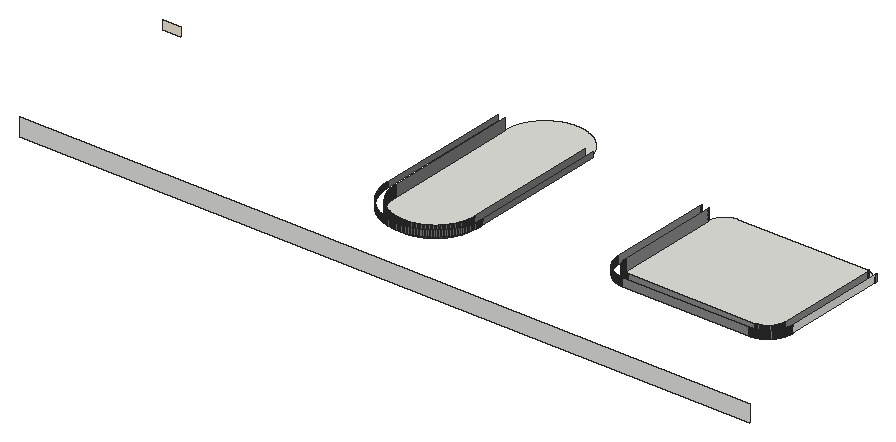
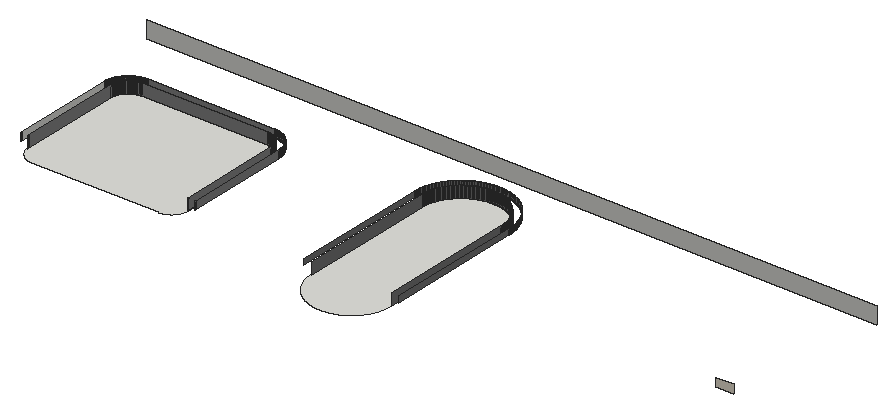
# SketchUp Ruby script. Lengths in inches.
U = 1.inch
M = Sketchup.active_model
def pt(a) = Geom::Point3d.new(a.map { |v| v * U })
def face(e, loops, mat)
  f = e.add_face(loops[0].map { |a| pt(a) })
  loops[1..].each { |l| e.add_face(l.map { |a| pt(a) }).erase! }
  f.material = f.back_material = mat if mat
  f
end
# faces: each face lists its corners as indices into pts; further lists are holes
def faces(e, pts, list, mat = nil) = list.each { |f| face(e, (f[0].is_a?(Array) ? f : [f]).map { |l| l.map { |i| pts[i] } }, mat) }
# xy, xz, yz: faces in a plane at the given z, y or x. An outline is a flat list of corners, or four numbers for a rectangle; further outlines are holes
def ring(l) = l.size == 4 ? [[l[0], l[1]], [l[2], l[1]], [l[2], l[3]], [l[0], l[3]]] : l.each_slice(2).to_a
def flat(e, list, mat, &to3) = list.each { |f| face(e, (f[0].is_a?(Array) ? f : [f]).map { |l| ring(l).map { |u, v| to3.(u, v) } }, mat) }
def xy(e, z, list, mat = nil) = flat(e, list, mat) { |x, y| [x, y, z] }
def xz(e, y, list, mat = nil) = flat(e, list, mat) { |x, z| [x, y, z] }
def yz(e, x, list, mat = nil) = flat(e, list, mat) { |y, z| [x, y, z] }
def lines(e, pts, list) = list.each { |a, b| e.add_line(pt(pts[a]), pt(pts[b])) }
# prism: a flat outline (further loops are holes) pulled along v
def prism(e, loops, v, mat = nil)
  f = face(e, loops, mat); d = Geom::Vector3d.new(v.map { |x| x * U })
  f.pushpull(f.normal.samedirection?(d) ? d.length : -d.length)
end
def box(e, o, s, mat = nil) = prism(e, [[o, [o[0] + s[0], o[1], o[2]], [o[0] + s[0], o[1] + s[1], o[2]], [o[0], o[1] + s[1], o[2]]]], [0, 0, s[2]], mat)
def at(x, y, z, deg = 0) = Geom::Transformation.translation(pt([x, y, z])) * Geom::Transformation.rotation(ORIGIN, Z_AXIS, deg.degrees)
def axes(o, x, y, z) = Geom::Transformation.new([*x, 0, *y, 0, *z, 0, *pt(o).to_a, 1])
def part(name) = M.definitions.add(name)
# library, detail: a bought-in or finely detailed component or shape, given as its bounding box
def library(name, o, s) = part(name).tap { |d| box(d.entities, o, s) }
def detail(e, o, s) = box(e.add_group.entities, o, s)
def put(e, d, t, mat = nil) = e.add_instance(d, t).tap { |i| i.material = mat if mat }
def group(e, t, mat = nil) = e.add_group.tap { |g| g.transformation = t; g.material = mat if mat }.entities
root = M.entities
M.materials.add("0027 AP L140 CRUSHED ICE").color = [241, 233, 217]
M.materials.add("[Slate Light Tile]").color = [119, 119, 119]
M.materials.add("[Stone Coursed Rough]").color = [137, 137, 137]
xy(root,-3,[[189,27,189.55,27.01,190.1,27.03,190.65,27.06,191.2,27.12,191.74,27.18,192.29,27.26,192.83,27.35,193.37,27.46,193.9,27.58,194.44,27.72,194.96,27.86,195.49,28.03,196.01,28.2,196.53,28.39,197.04,28.6,197.54,28.82,198.04,29.05,198.53,29.29,199.02,29.54,199.5,29.8125,199.97,30.09,200.4375,30.39,200.89,30.69,201.34,31.01,201.78,31.34,202.22,31.68,202.64,32.03,203.05,32.39,203.46,32.77,203.85,33.15,204.23,33.54,204.61,33.95,204.97,34.36,205.32,34.78,205.66,35.22,205.99,35.66,206.31,36.11,206.61,36.5625,206.91,37.03,207.1875,37.5,207.46,37.98,207.71,38.47,207.95,38.96,208.18,39.46,208.4,39.96,208.61,40.47,208.8,40.99,208.97,41.51,209.14,42.04,209.28,42.56,209.42,43.1,209.54,43.63,209.65,44.17,209.74,44.71,209.82,45.26,209.88,45.8,209.94,46.35,209.97,46.9,209.99,47.45,210,48,210,120,209.99,120.55,209.97,121.1,209.94,121.65,209.88,122.2,209.82,122.74,209.74,123.29,209.65,123.83,209.54,124.37,209.42,124.9,209.28,125.44,209.14,125.96,208.97,126.49,208.8,127.01,208.61,127.53,208.4,128.04,208.18,128.54,207.95,129.04,207.71,129.53,207.46,130.02,207.1875,130.5,206.91,130.97,206.61,131.4375,206.31,131.89,205.99,132.34,205.66,132.78,205.32,133.22,204.97,133.64,204.61,134.05,204.23,134.46,203.85,134.85,203.46,135.23,203.05,135.61,202.64,135.97,202.22,136.32,201.78,136.66,201.34,136.99,200.89,137.31,200.4375,137.61,199.97,137.91,199.5,138.1875,199.02,138.46,198.53,138.71,198.04,138.95,197.54,139.18,197.04,139.4,196.53,139.61,196.01,139.8,195.49,139.97,194.96,140.14,194.44,140.28,193.9,140.42,193.37,140.54,192.83,140.65,192.29,140.74,191.74,140.82,191.2,140.88,190.65,140.94,190.1,140.97,189.55,140.99,189,141,188.45,140.99,187.9,140.97,187.35,140.94,186.8,140.88,186.26,140.82,185.71,140.74,185.17,140.65,184.63,140.54,184.1,140.42,183.56,140.28,183.04,140.14,182.51,139.97,181.99,139.8,181.47,139.61,180.96,139.4,180.46,139.18,179.96,138.95,179.47,138.71,178.98,138.46,178.5,138.1875,178.03,137.91,177.5625,137.61,177.11,137.31,176.66,136.99,176.22,136.66,175.78,136.32,175.36,135.97,174.95,135.61,174.54,135.23,174.15,134.85,173.77,134.46,173.39,134.05,173.03,133.64,172.68,133.22,172.34,132.78,172.01,132.34,171.69,131.89,171.39,131.4375,171.09,130.97,170.8125,130.5,170.54,130.02,170.29,129.53,170.05,129.04,169.82,128.54,169.6,128.04,169.39,127.53,169.2,127.01,169.03,126.49,168.86,125.96,168.72,125.44,168.58,124.9,168.46,124.37,168.35,123.83,168.26,123.29,168.18,122.74,168.12,122.2,168.06,121.65,168.03,121.1,168.01,120.55,168,120,168,48,168.01,47.45,168.03,46.9,168.06,46.35,168.12,45.8,168.18,45.26,168.26,44.71,168.35,44.17,168.46,43.63,168.58,43.1,168.72,42.56,168.86,42.04,169.03,41.51,169.2,40.99,169.39,40.47,169.6,39.96,169.82,39.46,170.05,38.96,170.29,38.47,170.54,37.98,170.8125,37.5,171.09,37.03,171.39,36.5625,171.69,36.11,172.01,35.66,172.34,35.22,172.68,34.78,173.03,34.36,173.39,33.95,173.77,33.54,174.15,33.15,174.54,32.77,174.95,32.39,175.36,32.03,175.78,31.68,176.22,31.34,176.66,31.01,177.11,30.69,177.5625,30.39,178.03,30.09,178.5,29.8125,178.98,29.54,179.47,29.29,179.96,29.05,180.46,28.82,180.96,28.6,181.47,28.39,181.99,28.2,182.51,28.03,183.04,27.86,183.56,27.72,184.1,27.58,184.63,27.46,185.17,27.35,185.71,27.26,186.26,27.18,186.8,27.12,187.35,27.06,187.9,27.03,188.45,27.01]])
xy(root,-2,[[290.72,48,357.28,48,357.57,48.02,357.85,48.04,358.13,48.07,358.41,48.11,358.6875,48.16,358.96,48.22,359.24,48.28,359.78,48.44,360.05,48.53,360.3125,48.63,360.57,48.74,361.09,48.98,361.34,49.11,361.58,49.25,361.82,49.4,362.06,49.56,362.29,49.72,362.52,49.89,362.74,50.07,362.95,50.25,363.16,50.4375,363.36,50.64,363.5625,50.84,363.75,51.05,363.93,51.26,364.11,51.48,364.28,51.71,364.44,51.94,364.6,52.18,364.75,52.42,364.89,52.66,365.02,52.91,365.26,53.43,365.37,53.6875,365.47,53.95,365.56,54.22,365.72,54.76,365.78,55.04,365.84,55.3125,365.89,55.59,365.93,55.87,365.96,56.15,365.98,56.43,366,56.72,366,111.28,365.98,111.57,365.96,111.85,365.93,112.13,365.89,112.41,365.84,112.6875,365.78,112.96,365.72,113.24,365.56,113.78,365.47,114.05,365.37,114.3125,365.26,114.57,365.02,115.09,364.89,115.34,364.75,115.58,364.6,115.82,364.44,116.06,364.28,116.29,364.11,116.52,363.93,116.74,363.75,116.95,363.5625,117.16,363.36,117.36,363.16,117.5625,362.95,117.75,362.74,117.93,362.52,118.11,362.29,118.28,362.06,118.44,361.82,118.6,361.58,118.75,361.34,118.89,361.09,119.02,360.57,119.26,360.3125,119.37,360.05,119.47,359.78,119.56,359.24,119.72,358.96,119.78,358.6875,119.84,358.41,119.89,358.13,119.93,357.85,119.96,357.57,119.98,357.28,120,290.72,120,290.43,119.98,290.15,119.96,289.87,119.93,289.59,119.89,289.3125,119.84,289.04,119.78,288.76,119.72,288.22,119.56,287.95,119.47,287.6875,119.37,287.43,119.26,286.91,119.02,286.66,118.89,286.42,118.75,286.18,118.6,285.94,118.44,285.71,118.28,285.48,118.11,285.26,117.93,285.05,117.75,284.84,117.5625,284.64,117.36,284.4375,117.16,284.25,116.95,284.07,116.74,283.89,116.52,283.72,116.29,283.56,116.06,283.4,115.82,283.25,115.58,283.11,115.34,282.98,115.09,282.74,114.57,282.63,114.3125,282.53,114.05,282.44,113.78,282.28,113.24,282.22,112.96,282.16,112.6875,282.11,112.41,282.07,112.13,282.04,111.85,282.02,111.57,282,111.28,282,56.72,282.02,56.43,282.04,56.15,282.07,55.87,282.11,55.59,282.16,55.3125,282.22,55.04,282.28,54.76,282.44,54.22,282.53,53.95,282.63,53.6875,282.74,53.43,282.98,52.91,283.11,52.66,283.25,52.42,283.4,52.18,283.56,51.94,283.72,51.71,283.89,51.48,284.07,51.26,284.25,51.05,284.4375,50.84,284.64,50.64,284.84,50.4375,285.05,50.25,285.26,50.07,285.48,49.89,285.71,49.72,285.94,49.56,286.18,49.4,286.42,49.25,286.66,49.11,286.91,48.98,287.43,48.74,287.6875,48.63,287.95,48.53,288.22,48.44,288.76,48.28,289.04,48.22,289.3125,48.16,289.59,48.11,289.87,48.07,290.15,48.04,290.43,48.02]])
xz(root,0,[[9,-9,393,0]])
xz(root,44,[[291,0,357,4]],"[Stone Coursed Rough]")
xz(root,48,[[290.72,-2,291,4],[291,-2,357,4],[357,-2,357.28,4]],"[Stone Coursed Rough]")
xz(root,94,[[9,0,18,4.5]],"0027 AP L140 CRUSHED ICE")
yz(root,164,[[48,0,120,3]],"[Slate Light Tile]")
yz(root,168,[[48,-3,120,3]],"[Slate Light Tile]")
yz(root,210,[[48,-3,120,3]],"[Slate Light Tile]")
yz(root,214,[[48,0,120,3]],"[Slate Light Tile]")
yz(root,278,[[57,0,111,4]],"[Stone Coursed Rough]")
yz(root,282,[[56.72,-2,57,4],[57,-2,111,4],[111,-2,111.28,4]],"[Stone Coursed Rough]")
yz(root,366,[[56.72,-2,57,4],[57,-2,111,4],[111,-2,111.28,4]],"[Stone Coursed Rough]")
yz(root,370,[[57,0,111,4]])
p = [[187.35,27.06,-3],[187.35,27.06,3],[187.9,27.03,3],[187.9,27.03,-3],[188.45,27.01,3],[188.45,27.01,-3],
  [189,27,3],[189,27,-3],[189.55,27.01,3],[189.55,27.01,-3],[190.1,27.03,3],[190.1,27.03,-3],
  [190.65,27.06,3],[190.65,27.06,-3],[186.26,27.18,-3],[186.26,27.18,3],[186.8,27.12,3],[186.8,27.12,-3],
  [191.2,27.12,3],[191.2,27.12,-3],[191.74,27.18,3],[191.74,27.18,-3],[185.71,27.26,-3],[185.71,27.26,3],
  [192.29,27.26,3],[192.29,27.26,-3],[185.17,27.35,-3],[185.17,27.35,3],[192.83,27.35,3],[192.83,27.35,-3],
  [184.63,27.46,-3],[184.63,27.46,3],[193.37,27.46,3],[193.37,27.46,-3],[184.1,27.58,-3],[184.1,27.58,3],
  [193.9,27.58,3],[193.9,27.58,-3],[183.56,27.72,-3],[183.56,27.72,3],[194.44,27.72,3],[194.44,27.72,-3],
  [183.04,27.86,-3],[183.04,27.86,3],[194.96,27.86,3],[194.96,27.86,-3],[182.51,28.03,-3],[182.51,28.03,3],
  [195.49,28.03,3],[195.49,28.03,-3],[181.99,28.2,-3],[181.99,28.2,3],[196.01,28.2,3],[196.01,28.2,-3],
  [181.47,28.39,-3],[181.47,28.39,3],[196.53,28.39,3],[196.53,28.39,-3],[180.96,28.6,-3],[180.96,28.6,3],
  [197.04,28.6,3],[197.04,28.6,-3],[180.46,28.82,-3],[180.46,28.82,3],[197.54,28.82,3],[197.54,28.82,-3],
  [179.96,29.05,-3],[179.96,29.05,3],[198.04,29.05,3],[198.04,29.05,-3],[179.47,29.29,-3],[179.47,29.29,3],
  [198.53,29.29,3],[198.53,29.29,-3],[178.98,29.54,-3],[178.98,29.54,3],[199.02,29.54,3],[199.02,29.54,-3],
  [178.5,29.8125,-3],[178.5,29.8125,3],[199.5,29.8125,3],[199.5,29.8125,-3],[178.03,30.09,-3],[178.03,30.09,3],
  [199.97,30.09,3],[199.97,30.09,-3],[177.5625,30.39,-3],[177.5625,30.39,3],[200.4375,30.39,3],[200.4375,30.39,-3],
  [177.11,30.69,-3],[177.11,30.69,3],[200.89,30.69,3],[200.89,30.69,-3],[176.66,31.01,-3],[176.66,31.01,3],
  [201.34,31.01,3],[201.34,31.01,-3],[176.22,31.34,-3],[176.22,31.34,3],[201.78,31.34,3],[201.78,31.34,-3],
  [175.78,31.68,-3],[175.78,31.68,3],[202.22,31.68,3],[202.22,31.68,-3],[175.36,32.03,-3],[175.36,32.03,3],
  [202.64,32.03,3],[202.64,32.03,-3],[174.95,32.39,-3],[174.95,32.39,3],[203.05,32.39,3],[203.05,32.39,-3],
  [174.54,32.77,-3],[174.54,32.77,3],[203.46,32.77,3],[203.46,32.77,-3],[174.15,33.15,-3],[174.15,33.15,3],
  [203.85,33.15,3],[203.85,33.15,-3],[173.77,33.54,-3],[173.77,33.54,3],[204.23,33.54,3],[204.23,33.54,-3],
  [173.39,33.95,-3],[173.39,33.95,3],[204.61,33.95,3],[204.61,33.95,-3],[173.03,34.36,-3],[173.03,34.36,3],
  [204.97,34.36,3],[204.97,34.36,-3],[172.68,34.78,-3],[172.68,34.78,3],[205.32,34.78,3],[205.32,34.78,-3],
  [172.34,35.22,-3],[172.34,35.22,3],[205.66,35.22,3],[205.66,35.22,-3],[172.01,35.66,-3],[172.01,35.66,3],
  [205.99,35.66,3],[205.99,35.66,-3],[171.69,36.11,-3],[171.69,36.11,3],[206.31,36.11,3],[206.31,36.11,-3],
  [171.39,36.5625,-3],[171.39,36.5625,3],[206.61,36.5625,3],[206.61,36.5625,-3],[171.09,37.03,-3],[171.09,37.03,3],
  [206.91,37.03,3],[206.91,37.03,-3],[170.8125,37.5,-3],[170.8125,37.5,3],[207.1875,37.5,3],[207.1875,37.5,-3],
  [170.54,37.98,-3],[170.54,37.98,3],[207.46,37.98,3],[207.46,37.98,-3],[170.29,38.47,-3],[170.29,38.47,3],
  [207.71,38.47,3],[207.71,38.47,-3],[170.05,38.96,-3],[170.05,38.96,3],[207.95,38.96,3],[207.95,38.96,-3],
  [169.82,39.46,-3],[169.82,39.46,3],[208.18,39.46,3],[208.18,39.46,-3],[169.6,39.96,-3],[169.6,39.96,3],
  [208.4,39.96,3],[208.4,39.96,-3],[169.39,40.47,-3],[169.39,40.47,3],[208.61,40.47,3],[208.61,40.47,-3],
  [169.2,40.99,-3],[169.2,40.99,3],[208.8,40.99,3],[208.8,40.99,-3],[169.03,41.51,-3],[169.03,41.51,3],
  [208.97,41.51,3],[208.97,41.51,-3],[168.86,42.04,-3],[168.86,42.04,3],[209.14,42.04,3],[209.14,42.04,-3],
  [168.72,42.56,-3],[168.72,42.56,3],[209.28,42.56,3],[209.28,42.56,-3],[168.58,43.1,-3],[168.58,43.1,3],
  [209.42,43.1,3],[209.42,43.1,-3],[168.46,43.63,-3],[168.46,43.63,3],[209.54,43.63,3],[209.54,43.63,-3],
  [168.35,44.17,-3],[168.35,44.17,3],[209.65,44.17,3],[209.65,44.17,-3],[168.26,44.71,-3],[168.26,44.71,3],
  [209.74,44.71,3],[209.74,44.71,-3],[168.18,45.26,-3],[168.18,45.26,3],[209.82,45.26,3],[209.82,45.26,-3],
  [168.12,45.8,-3],[168.12,45.8,3],[209.88,45.8,3],[209.88,45.8,-3],[168.06,46.35,-3],[168.06,46.35,3],
  [209.94,46.35,3],[209.94,46.35,-3],[168.03,46.9,-3],[168.03,46.9,3],[209.97,46.9,3],[209.97,46.9,-3],
  [168.01,47.45,-3],[168.01,47.45,3],[209.99,47.45,3],[209.99,47.45,-3],[168,48,-3],[168,48,3],
  [210,48,3],[210,48,-3],[290.15,48.04,-2],[289.87,48.07,-2],[289.87,48.07,4],[290.15,48.04,4],
  [290.43,48.02,-2],[290.43,48.02,4],[290.72,48,-2],[290.72,48,4],[357.57,48.02,-2],[357.28,48,-2],
  [357.28,48,4],[357.57,48.02,4],[357.85,48.04,-2],[357.85,48.04,4],[358.13,48.07,-2],[358.13,48.07,4],
  [289.59,48.11,-2],[289.3125,48.16,-2],[289.3125,48.16,4],[289.59,48.11,4],[358.41,48.11,-2],[358.41,48.11,4],
  [358.6875,48.16,-2],[358.6875,48.16,4],[289.04,48.22,-2],[288.76,48.28,-2],[288.76,48.28,4],[289.04,48.22,4],
  [358.96,48.22,-2],[358.96,48.22,4],[359.24,48.28,-2],[359.24,48.28,4],[288.49,48.36,-2],[288.49,48.36,4],
  [359.51,48.36,-2],[359.51,48.36,4],[288.22,48.44,-2],[287.95,48.53,-2],[287.95,48.53,4],[288.22,48.44,4],
  [359.78,48.44,-2],[359.78,48.44,4],[360.05,48.53,-2],[360.05,48.53,4],[287.6875,48.63,-2],[287.6875,48.63,4],
  [360.3125,48.63,-2],[360.3125,48.63,4],[287.43,48.74,-2],[287.43,48.74,4],[360.57,48.74,-2],[360.57,48.74,4],
  [287.17,48.86,-2],[287.17,48.86,4],[360.83,48.86,-2],[360.83,48.86,4],[286.91,48.98,-2],[286.91,48.98,4],
  [361.09,48.98,-2],[361.09,48.98,4],[286.66,49.11,-2],[286.66,49.11,4],[361.34,49.11,-2],[361.34,49.11,4],
  [286.42,49.25,-2],[286.42,49.25,4],[361.58,49.25,-2],[361.58,49.25,4],[286.18,49.4,-2],[286.18,49.4,4],
  [361.82,49.4,-2],[361.82,49.4,4],[285.94,49.56,-2],[285.94,49.56,4],[362.06,49.56,-2],[362.06,49.56,4],
  [285.71,49.72,-2],[285.71,49.72,4],[362.29,49.72,-2],[362.29,49.72,4],[285.48,49.89,-2],[285.48,49.89,4],
  [362.52,49.89,-2],[362.52,49.89,4],[285.26,50.07,-2],[285.26,50.07,4],[362.74,50.07,-2],[362.74,50.07,4],
  [285.05,50.25,-2],[285.05,50.25,4],[362.95,50.25,-2],[362.95,50.25,4],[284.84,50.4375,-2],[284.84,50.4375,4],
  [363.16,50.4375,-2],[363.16,50.4375,4],[284.64,50.64,-2],[284.64,50.64,4],[363.36,50.64,-2],[363.36,50.64,4],
  [284.4375,50.84,-2],[284.4375,50.84,4],[363.5625,50.84,-2],[363.5625,50.84,4],[284.25,51.05,-2],[284.25,51.05,4],
  [363.75,51.05,-2],[363.75,51.05,4],[284.07,51.26,-2],[284.07,51.26,4],[363.93,51.26,-2],[363.93,51.26,4],
  [283.89,51.48,-2],[283.89,51.48,4],[364.11,51.48,-2],[364.11,51.48,4],[283.72,51.71,-2],[283.72,51.71,4],
  [364.28,51.71,-2],[364.28,51.71,4],[283.56,51.94,-2],[283.56,51.94,4],[364.44,51.94,-2],[364.44,51.94,4],
  [283.4,52.18,-2],[283.4,52.18,4],[364.6,52.18,-2],[364.6,52.18,4],[283.25,52.42,-2],[283.25,52.42,4],
  [364.75,52.42,-2],[364.75,52.42,4],[283.11,52.66,-2],[283.11,52.66,4],[364.89,52.66,-2],[364.89,52.66,4],
  [282.98,52.91,-2],[282.98,52.91,4],[365.02,52.91,-2],[365.02,52.91,4],[282.86,53.17,-2],[282.86,53.17,4],
  [365.14,53.17,-2],[365.14,53.17,4],[282.74,53.43,-2],[282.74,53.43,4],[365.26,53.43,-2],[365.26,53.43,4],
  [282.63,53.6875,-2],[282.63,53.6875,4],[365.37,53.6875,-2],[365.37,53.6875,4],[282.53,53.95,-2],[282.53,53.95,4],
  [365.47,53.95,-2],[365.47,53.95,4],[282.44,54.22,-2],[282.44,54.22,4],[365.56,54.22,-2],[365.56,54.22,4],
  [282.36,54.49,-2],[282.36,54.49,4],[365.64,54.49,-2],[365.64,54.49,4],[282.28,54.76,-2],[282.28,54.76,4],
  [365.72,54.76,-2],[365.72,54.76,4],[282.22,55.04,-2],[282.22,55.04,4],[365.78,55.04,-2],[365.78,55.04,4],
  [282.16,55.3125,-2],[282.16,55.3125,4],[365.84,55.3125,-2],[365.84,55.3125,4],[282.11,55.59,-2],[282.11,55.59,4],
  [365.89,55.59,-2],[365.89,55.59,4],[282.07,55.87,-2],[282.07,55.87,4],[365.93,55.87,-2],[365.93,55.87,4],
  [282.04,56.15,-2],[282.04,56.15,4],[365.96,56.15,-2],[365.96,56.15,4],[282.02,56.43,-2],[282.02,56.43,4],
  [365.98,56.43,-2],[365.98,56.43,4],[282,56.72,-2],[282,56.72,4],[366,56.72,-2],[366,56.72,4],
  [282,111.28,-2],[282.02,111.57,-2],[282.02,111.57,4],[282,111.28,4],[365.98,111.57,-2],[366,111.28,-2],
  [366,111.28,4],[365.98,111.57,4],[282.04,111.85,-2],[282.04,111.85,4],[365.96,111.85,-2],[365.96,111.85,4],
  [365.93,112.13,-2],[365.93,112.13,4],[187.04,23.08,0],[187.69,23.03,0],[187.69,23.03,3],[187.04,23.08,3],
  [188.35,23.01,0],[188.35,23.01,3],[189,23,0],[189,23,3],[189.65,23.01,0],[189.65,23.01,3],
  [190.31,23.03,0],[190.31,23.03,3],[190.96,23.08,0],[190.96,23.08,3],[185.74,23.21,0],[186.39,23.14,0],
  [186.39,23.14,3],[185.74,23.21,3],[191.61,23.14,0],[191.61,23.14,3],[192.26,23.21,0],[192.26,23.21,3],
  [185.09,23.31,0],[185.09,23.31,3],[192.91,23.31,0],[192.91,23.31,3],[184.44,23.42,0],[184.44,23.42,3],
  [193.56,23.42,0],[193.56,23.42,3],[183.8,23.55,0],[183.8,23.55,3],[194.2,23.55,0],[194.2,23.55,3],
  [183.16,23.69,0],[183.16,23.69,3],[194.84,23.69,0],[194.84,23.69,3],[182.53,23.85,0],[182.53,23.85,3],
  [195.47,23.85,0],[195.47,23.85,3],[181.9,24.03,0],[181.9,24.03,3],[196.1,24.03,0],[196.1,24.03,3],
  [181.27,24.22,0],[181.27,24.22,3],[196.73,24.22,0],[196.73,24.22,3],[180.65,24.43,0],[180.65,24.43,3],
  [197.35,24.43,0],[197.35,24.43,3],[180.04,24.66,0],[180.04,24.66,3],[197.96,24.66,0],[197.96,24.66,3],
  [179.43,24.9,0],[179.43,24.9,3],[198.57,24.9,0],[198.57,24.9,3],[178.83,25.16,0],[178.83,25.16,3],
  [199.17,25.16,0],[199.17,25.16,3],[178.24,25.44,0],[178.24,25.44,3],[199.76,25.44,0],[199.76,25.44,3],
  [177.65,25.72,0],[177.65,25.72,3],[200.35,25.72,0],[200.35,25.72,3],[177.07,26.03,0],[177.07,26.03,3],
  [200.93,26.03,0],[200.93,26.03,3],[176.5,26.35,0],[176.5,26.35,3],[201.5,26.35,0],[201.5,26.35,3],
  [175.9375,26.68,0],[175.9375,26.68,3],[202.0625,26.68,0],[202.0625,26.68,3],[175.38,27.03,0],[175.38,27.03,3],
  [202.62,27.03,0],[202.62,27.03,3],[174.84,27.4,0],[174.84,27.4,3],[203.16,27.4,0],[203.16,27.4,3],
  [174.31,27.77,0],[174.31,27.77,3],[203.69,27.77,0],[203.69,27.77,3],[173.78,28.17,0],[173.78,28.17,3],
  [204.22,28.17,0],[204.22,28.17,3],[173.27,28.57,0],[173.27,28.57,3],[204.73,28.57,0],[204.73,28.57,3],
  [172.76,28.99,0],[172.76,28.99,3],[205.24,28.99,0],[205.24,28.99,3],[172.27,29.42,0],[172.27,29.42,3],
  [205.73,29.42,0],[205.73,29.42,3],[171.79,29.87,0],[171.79,29.87,3],[206.21,29.87,0],[206.21,29.87,3],
  [171.32,30.32,0],[171.32,30.32,3],[206.68,30.32,0],[206.68,30.32,3],[170.87,30.79,0],[170.87,30.79,3],
  [207.13,30.79,0],[207.13,30.79,3],[170.42,31.27,0],[170.42,31.27,3],[207.58,31.27,0],[207.58,31.27,3],
  [169.99,31.76,0],[169.99,31.76,3],[208.01,31.76,0],[208.01,31.76,3],[169.57,32.27,0],[169.57,32.27,3],
  [208.43,32.27,0],[208.43,32.27,3],[169.17,32.78,0],[169.17,32.78,3],[208.83,32.78,0],[208.83,32.78,3],
  [168.77,33.31,0],[168.77,33.31,3],[209.23,33.31,0],[209.23,33.31,3],[168.4,33.84,0],[168.4,33.84,3],
  [209.6,33.84,0],[209.6,33.84,3],[168.03,34.38,0],[168.03,34.38,3],[209.97,34.38,0],[209.97,34.38,3],
  [167.68,34.9375,0],[167.68,34.9375,3],[210.32,34.9375,0],[210.32,34.9375,3],[167.35,35.5,0],[167.35,35.5,3],
  [210.65,35.5,0],[210.65,35.5,3],[167.03,36.07,0],[167.03,36.07,3],[210.97,36.07,0],[210.97,36.07,3],
  [166.72,36.65,0],[166.72,36.65,3],[211.28,36.65,0],[211.28,36.65,3],[166.44,37.24,0],[166.44,37.24,3],
  [211.56,37.24,0],[211.56,37.24,3],[166.16,37.83,0],[166.16,37.83,3],[211.84,37.83,0],[211.84,37.83,3],
  [165.9,38.43,0],[165.9,38.43,3],[212.1,38.43,0],[212.1,38.43,3],[165.66,39.04,0],[165.66,39.04,3],
  [212.34,39.04,0],[212.34,39.04,3],[165.43,39.65,0],[165.43,39.65,3],[212.57,39.65,0],[212.57,39.65,3],
  [165.22,40.27,0],[165.22,40.27,3],[212.78,40.27,0],[212.78,40.27,3],[165.03,40.9,0],[165.03,40.9,3],
  [212.97,40.9,0],[212.97,40.9,3],[164.85,41.53,0],[164.85,41.53,3],[213.15,41.53,0],[213.15,41.53,3],
  [164.69,42.16,0],[164.69,42.16,3],[213.31,42.16,0],[213.31,42.16,3],[164.55,42.8,0],[164.55,42.8,3],
  [213.45,42.8,0],[213.45,42.8,3],[164.42,43.44,0],[164.42,43.44,3],[213.58,43.44,0],[213.58,43.44,3],
  [164.31,44.09,0],[164.31,44.09,3],[213.69,44.09,0],[213.69,44.09,3],[289.78,44.06,0],[290.18,44.03,0],
  [290.18,44.03,4],[289.78,44.06,4],[290.59,44.01,0],[290.59,44.01,4],[291,44,0],[291,44,4],
  [357,44,0],[357.41,44.01,0],[357.41,44.01,4],[357,44,4],[357.82,44.03,0],[357.82,44.03,4],
  [358.22,44.06,0],[358.22,44.06,4],[164.21,44.74,0],[164.21,44.74,3],[213.79,44.74,0],[213.79,44.74,3],
  [288.97,44.16,0],[289.37,44.1,0],[289.37,44.1,4],[288.97,44.16,4],[358.63,44.1,0],[358.63,44.1,4],
  [359.03,44.16,0],[359.03,44.16,4],[288.16,44.3125,0],[288.5625,44.23,0],[288.5625,44.23,4],[288.16,44.3125,4],
  [359.4375,44.23,0],[359.4375,44.23,4],[359.84,44.3125,0],[359.84,44.3125,4],[287.77,44.41,0],[287.77,44.41,4],
  [360.23,44.41,0],[360.23,44.41,4],[287.375,44.52,0],[287.375,44.52,4],[360.625,44.52,0],[360.625,44.52,4],
  [286.98,44.64,0],[286.98,44.64,4],[361.02,44.64,0],[361.02,44.64,4],[286.6,44.77,0],[286.6,44.77,4],
  [361.4,44.77,0],[361.4,44.77,4],[164.14,45.39,0],[164.14,45.39,3],[213.86,45.39,0],[213.86,45.39,3],
  [286.21,44.91,0],[286.21,44.91,4],[361.79,44.91,0],[361.79,44.91,4],[285.84,45.07,0],[285.84,45.07,4],
  [362.16,45.07,0],[362.16,45.07,4],[285.46,45.24,0],[285.46,45.24,4],[362.54,45.24,0],[362.54,45.24,4],
  [285.1,45.42,0],[285.1,45.42,4],[362.9,45.42,0],[362.9,45.42,4],[164.08,46.04,0],[164.08,46.04,3],
  [213.92,46.04,0],[213.92,46.04,3],[284.74,45.61,0],[284.74,45.61,4],[363.26,45.61,0],[363.26,45.61,4],
  [284.38,45.81,0],[284.38,45.81,4],[363.62,45.81,0],[363.62,45.81,4],[284.03,46.02,0],[284.03,46.02,4],
  [363.97,46.02,0],[363.97,46.02,4],[164.03,46.69,0],[164.03,46.69,3],[213.97,46.69,0],[213.97,46.69,3],
  [283.69,46.25,0],[283.69,46.25,4],[364.31,46.25,0],[364.31,46.25,4],[283.36,46.48,0],[283.36,46.48,4],
  [364.64,46.48,0],[364.64,46.48,4],[283.03,46.73,0],[283.03,46.73,4],[364.97,46.73,0],[364.97,46.73,4],
  [164.01,47.35,0],[164.01,47.35,3],[213.99,47.35,0],[213.99,47.35,3],[282.71,46.98,0],[282.71,46.98,4],
  [365.29,46.98,0],[365.29,46.98,4],[282.4,47.25,0],[282.4,47.25,4],[365.6,47.25,0],[365.6,47.25,4],
  [282.1,47.52,0],[282.1,47.52,4],[365.9,47.52,0],[365.9,47.52,4],[164,48,0],[164,48,3],
  [214,48,0],[214,48,3],[281.81,47.81,0],[281.81,47.81,4],[366.19,47.81,0],[366.19,47.81,4],
  [281.52,48.1,0],[281.52,48.1,4],[366.48,48.1,0],[366.48,48.1,4],[281.25,48.4,0],[281.25,48.4,4],
  [366.75,48.4,0],[366.75,48.4,4],[280.98,48.71,0],[280.98,48.71,4],[367.02,48.71,0],[367.02,48.71,4],
  [280.73,49.03,0],[280.73,49.03,4],[367.27,49.03,0],[367.27,49.03,4],[280.48,49.36,0],[280.48,49.36,4],
  [367.52,49.36,0],[367.52,49.36,4],[280.25,49.69,0],[280.25,49.69,4],[367.75,49.69,0],[367.75,49.69,4],
  [280.02,50.03,0],[280.02,50.03,4],[367.98,50.03,0],[367.98,50.03,4],[279.81,50.38,0],[279.81,50.38,4],
  [368.19,50.38,0],[368.19,50.38,4],[279.61,50.74,0],[279.61,50.74,4],[368.39,50.74,0],[368.39,50.74,4],
  [279.42,51.1,0],[279.42,51.1,4],[368.58,51.1,0],[368.58,51.1,4],[279.24,51.46,0],[279.24,51.46,4],
  [368.76,51.46,0],[368.76,51.46,4],[279.07,51.84,0],[279.07,51.84,4],[368.93,51.84,0],[368.93,51.84,4],
  [278.91,52.21,0],[278.91,52.21,4],[369.09,52.21,0],[369.09,52.21,4],[278.77,52.6,0],[278.77,52.6,4],
  [369.23,52.6,0],[369.23,52.6,4],[278.64,52.98,0],[278.64,52.98,4],[369.36,52.98,0],[369.36,52.98,4],
  [278.52,53.375,0],[278.52,53.375,4],[369.48,53.375,0],[369.48,53.375,4],[278.41,53.77,0],[278.41,53.77,4],
  [369.59,53.77,0],[369.59,53.77,4],[278.3125,54.16,0],[278.3125,54.16,4],[369.6875,54.16,0],[369.6875,54.16,4],
  [278.23,54.5625,0],[278.23,54.5625,4],[369.77,54.5625,0],[369.77,54.5625,4],[278.16,54.97,0],[278.16,54.97,4],
  [369.84,54.97,0],[369.84,54.97,4],[278.1,55.37,0],[278.1,55.37,4],[369.9,55.37,0],[369.9,55.37,4],
  [278.06,55.78,0],[278.06,55.78,4],[369.94,55.78,0],[369.94,55.78,4],[278.03,56.18,0],[278.03,56.18,4],
  [369.97,56.18,0],[369.97,56.18,4],[278.01,56.59,0],[278.01,56.59,4],[369.99,56.59,0],[369.99,56.59,4],
  [278,57,0],[278,57,4],[370,57,0],[370,57,4],[278.01,111.41,0],[278,111,0],
  [278,111,4],[278.01,111.41,4],[370,111,0],[369.99,111.41,0],[369.99,111.41,4],[370,111,4],
  [278.03,111.82,0],[278.03,111.82,4],[369.97,111.82,0],[369.97,111.82,4]]
faces(root,p,[[0,1,2,3],[3,2,4,5],[5,4,6,7],[7,6,8,9],[9,8,10,11],[11,10,12,13],[14,15,16,17],[17,16,1,0],
  [13,12,18,19],[19,18,20,21],[22,23,15,14],[21,20,24,25],[26,27,23,22],[25,24,28,29],[30,31,27,26],[29,28,32,33],
  [34,35,31,30],[33,32,36,37],[38,39,35,34],[37,36,40,41],[42,43,39,38],[41,40,44,45],[46,47,43,42],[45,44,48,49],
  [50,51,47,46],[49,48,52,53],[54,55,51,50],[53,52,56,57],[58,59,55,54],[57,56,60,61],[62,63,59,58],[61,60,64,65],
  [66,67,63,62],[65,64,68,69],[70,71,67,66],[69,68,72,73],[74,75,71,70],[73,72,76,77],[78,79,75,74],[77,76,80,81],
  [82,83,79,78],[81,80,84,85],[86,87,83,82],[85,84,88,89],[90,91,87,86],[89,88,92,93],[94,95,91,90],[93,92,96,97],
  [98,99,95,94],[97,96,100,101],[102,103,99,98],[101,100,104,105],[106,107,103,102],[105,104,108,109],[110,111,107,106],[109,108,112,113],
  [114,115,111,110],[113,112,116,117],[118,119,115,114],[117,116,120,121],[122,123,119,118],[121,120,124,125],[126,127,123,122],[125,124,128,129],
  [130,131,127,126],[129,128,132,133],[134,135,131,130],[133,132,136,137],[138,139,135,134],[137,136,140,141],[142,143,139,138],[141,140,144,145],
  [146,147,143,142],[145,144,148,149],[150,151,147,146],[149,148,152,153],[154,155,151,150],[153,152,156,157],[158,159,155,154],[157,156,160,161],
  [162,163,159,158],[161,160,164,165],[166,167,163,162],[165,164,168,169],[170,171,167,166],[169,168,172,173],[174,175,171,170],[173,172,176,177],
  [178,179,175,174],[177,176,180,181],[182,183,179,178],[181,180,184,185],[186,187,183,182],[185,184,188,189],[190,191,187,186],[189,188,192,193],
  [194,195,191,190],[193,192,196,197],[198,199,195,194],[197,196,200,201],[202,203,199,198],[201,200,204,205],[206,207,203,202],[205,204,208,209],
  [210,211,207,206],[209,208,212,213],[214,215,211,210],[213,212,216,217],[218,219,215,214],[217,216,220,221],[222,223,219,218],[221,220,224,225],
  [226,227,223,222],[225,224,228,229],[230,231,227,226],[229,228,232,233],[234,235,231,230],[233,232,236,237],[238,239,235,234],[237,236,240,241],
  [452,453,454,455],[453,456,457,454],[456,458,459,457],[458,460,461,459],[460,462,463,461],[462,464,465,463],[466,467,468,469],[467,452,455,468],
  [464,470,471,465],[470,472,473,471],[474,466,469,475],[472,476,477,473],[478,474,475,479],[476,480,481,477],[482,478,479,483],[480,484,485,481],
  [486,482,483,487],[484,488,489,485],[490,486,487,491],[488,492,493,489],[494,490,491,495],[492,496,497,493],[498,494,495,499],[496,500,501,497],
  [502,498,499,503],[500,504,505,501],[506,502,503,507],[504,508,509,505],[510,506,507,511],[508,512,513,509],[514,510,511,515],[512,516,517,513],
  [518,514,515,519],[516,520,521,517],[522,518,519,523],[520,524,525,521],[526,522,523,527],[524,528,529,525],[530,526,527,531],[528,532,533,529],
  [534,530,531,535],[532,536,537,533],[538,534,535,539],[536,540,541,537],[542,538,539,543],[540,544,545,541],[546,542,543,547],[544,548,549,545],
  [550,546,547,551],[548,552,553,549],[554,550,551,555],[552,556,557,553],[558,554,555,559],[556,560,561,557],[562,558,559,563],[560,564,565,561],
  [566,562,563,567],[564,568,569,565],[570,566,567,571],[568,572,573,569],[574,570,571,575],[572,576,577,573],[578,574,575,579],[576,580,581,577],
  [582,578,579,583],[580,584,585,581],[586,582,583,587],[584,588,589,585],[590,586,587,591],[588,592,593,589],[594,590,591,595],[592,596,597,593],
  [598,594,595,599],[596,600,601,597],[602,598,599,603],[600,604,605,601],[606,602,603,607],[604,608,609,605],[610,606,607,611],[608,612,613,609],
  [614,610,611,615],[612,616,617,613],[618,614,615,619],[616,620,621,617],[622,618,619,623],[620,624,625,621],[626,622,623,627],[624,628,629,625],
  [630,626,627,631],[628,632,633,629],[634,630,631,635],[632,636,637,633],[638,634,635,639],[636,640,641,637],[642,638,639,643],[640,644,645,641],
  [646,642,643,647],[644,648,649,645],[650,646,647,651],[648,652,653,649],[654,650,651,655],[652,656,657,653],[658,654,655,659],[656,660,661,657],
  [662,658,659,663],[660,664,665,661],[666,662,663,667],[664,668,669,665],[686,666,667,687],[668,688,689,669],[722,686,687,723],[688,724,725,689],
  [742,722,723,743],[724,744,745,725],[758,742,743,759],[744,760,761,745],[774,758,759,775],[760,776,777,761],[790,774,775,791],[776,792,793,777]],"[Slate Light Tile]")
faces(root,p,[[242,243,244,245],[246,242,245,247],[248,246,247,249],[250,251,252,253],[254,250,253,255],[256,254,255,257],[258,259,260,261],[243,258,261,244],
  [262,256,257,263],[264,262,263,265],[266,267,268,269],[259,266,269,260],[270,264,265,271],[272,270,271,273],[267,274,275,268],[276,272,273,277],
  [278,279,280,281],[274,278,281,275],[282,276,277,283],[284,282,283,285],[279,286,287,280],[288,284,285,289],[286,290,291,287],[292,288,289,293],
  [290,294,295,291],[296,292,293,297],[294,298,299,295],[300,296,297,301],[298,302,303,299],[304,300,301,305],[302,306,307,303],[308,304,305,309],
  [306,310,311,307],[312,308,309,313],[310,314,315,311],[316,312,313,317],[314,318,319,315],[320,316,317,321],[318,322,323,319],[324,320,321,325],
  [322,326,327,323],[328,324,325,329],[326,330,331,327],[332,328,329,333],[330,334,335,331],[336,332,333,337],[334,338,339,335],[340,336,337,341],
  [338,342,343,339],[344,340,341,345],[342,346,347,343],[348,344,345,349],[346,350,351,347],[352,348,349,353],[350,354,355,351],[356,352,353,357],
  [354,358,359,355],[360,356,357,361],[358,362,363,359],[364,360,361,365],[362,366,367,363],[368,364,365,369],[366,370,371,367],[372,368,369,373],
  [370,374,375,371],[376,372,373,377],[374,378,379,375],[380,376,377,381],[378,382,383,379],[384,380,381,385],[382,386,387,383],[388,384,385,389],
  [386,390,391,387],[392,388,389,393],[390,394,395,391],[396,392,393,397],[394,398,399,395],[400,396,397,401],[398,402,403,399],[404,400,401,405],
  [402,406,407,403],[408,404,405,409],[406,410,411,407],[412,408,409,413],[410,414,415,411],[416,412,413,417],[414,418,419,415],[420,416,417,421],
  [418,422,423,419],[424,420,421,425],[422,426,427,423],[428,424,425,429],[426,430,431,427],[432,428,429,433],[430,434,435,431],[436,432,433,437],
  [438,439,440,441],[442,443,444,445],[439,446,447,440],[448,442,445,449],[450,448,449,451],[670,671,672,673],[671,674,675,672],[674,676,677,675],
  [678,679,680,681],[679,682,683,680],[682,684,685,683],[690,691,692,693],[691,670,673,692],[684,694,695,685],[694,696,697,695],[698,699,700,701],
  [699,690,693,700],[696,702,703,697],[702,704,705,703],[706,698,701,707],[704,708,709,705],[710,706,707,711],[708,712,713,709],[714,710,711,715],
  [712,716,717,713],[718,714,715,719],[716,720,721,717],[726,718,719,727],[720,728,729,721],[730,726,727,731],[728,732,733,729],[734,730,731,735],
  [732,736,737,733],[738,734,735,739],[736,740,741,737],[746,738,739,747],[740,748,749,741],[750,746,747,751],[748,752,753,749],[754,750,751,755],
  [752,756,757,753],[762,754,755,763],[756,764,765,757],[766,762,763,767],[764,768,769,765],[770,766,767,771],[768,772,773,769],[778,770,771,779],
  [772,780,781,773],[782,778,779,783],[780,784,785,781],[786,782,783,787],[784,788,789,785],[794,786,787,795],[788,796,797,789],[798,794,795,799],
  [796,800,801,797],[802,798,799,803],[800,804,805,801],[806,802,803,807],[804,808,809,805],[810,806,807,811],[808,812,813,809],[814,810,811,815],
  [812,816,817,813],[818,814,815,819],[816,820,821,817],[822,818,819,823],[820,824,825,821],[826,822,823,827],[824,828,829,825],[830,826,827,831],
  [828,832,833,829],[834,830,831,835],[832,836,837,833],[838,834,835,839],[836,840,841,837],[842,838,839,843],[840,844,845,841],[846,842,843,847],
  [844,848,849,845],[850,846,847,851],[848,852,853,849],[854,850,851,855],[852,856,857,853],[858,854,855,859],[856,860,861,857],[862,858,859,863],
  [860,864,865,861],[866,862,863,867],[864,868,869,865],[870,866,867,871],[868,872,873,869],[874,870,871,875],[872,876,877,873],[878,874,875,879],
  [876,880,881,877],[882,878,879,883],[880,884,885,881],[886,882,883,887],[884,888,889,885],[890,886,887,891],[888,892,893,889],[894,890,891,895],
  [892,896,897,893],[898,899,900,901],[902,903,904,905],[906,898,901,907],[903,908,909,904]],"[Stone Coursed Rough]")
